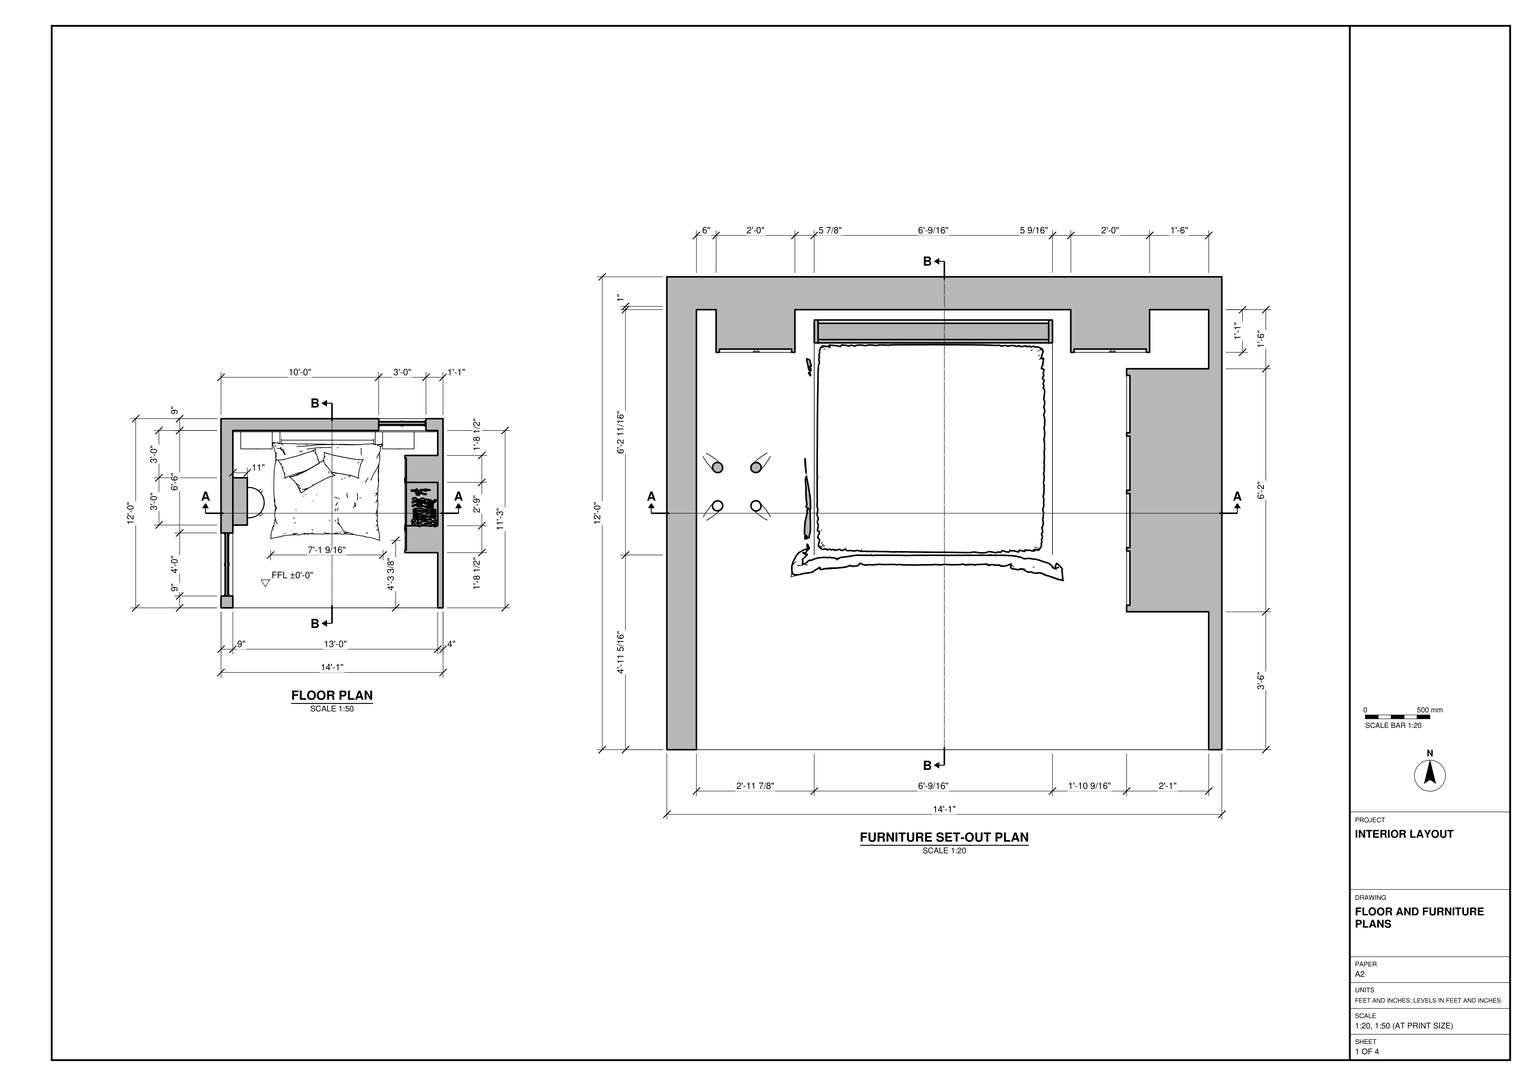
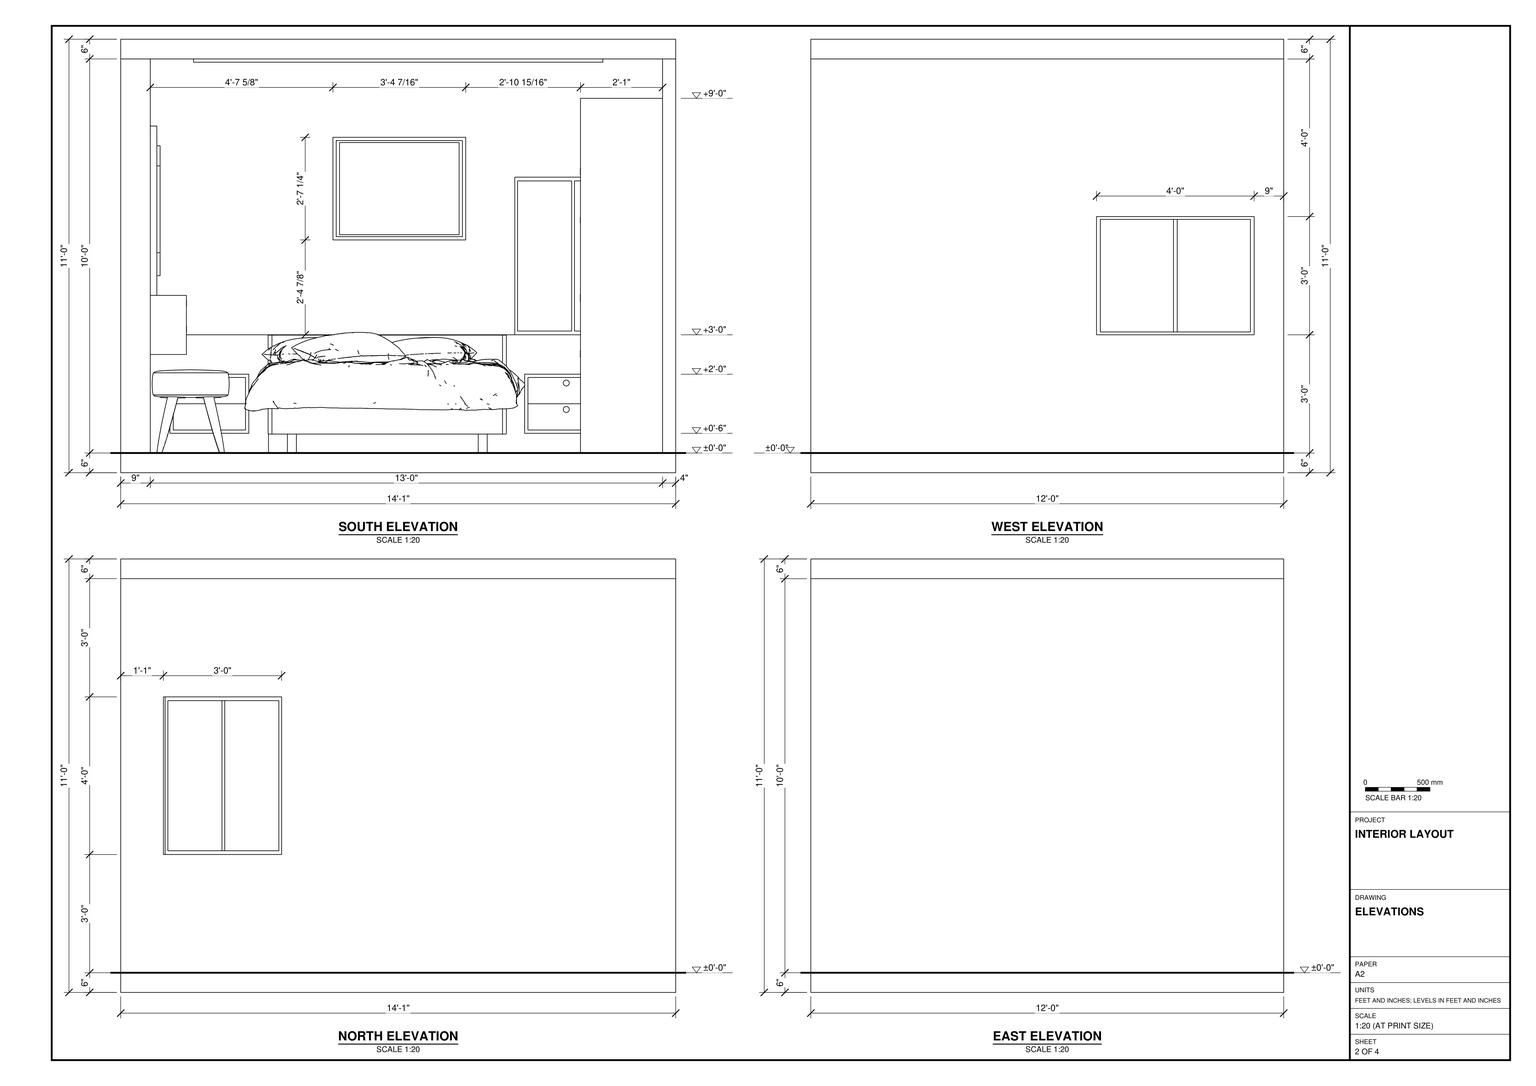
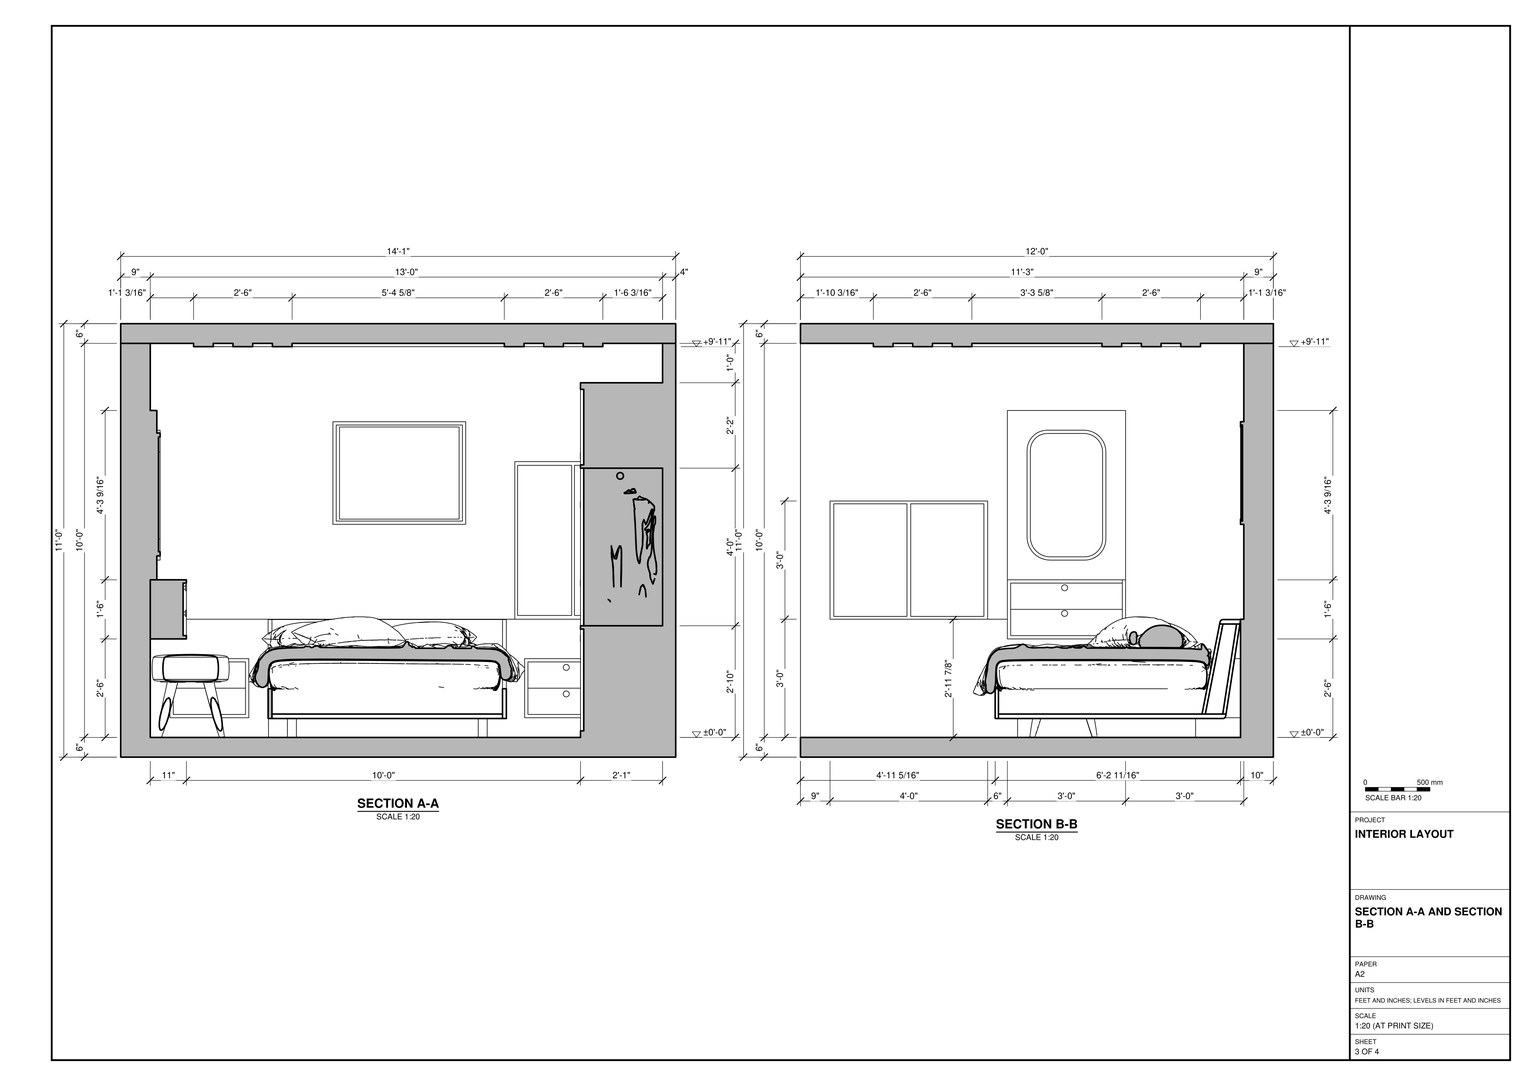
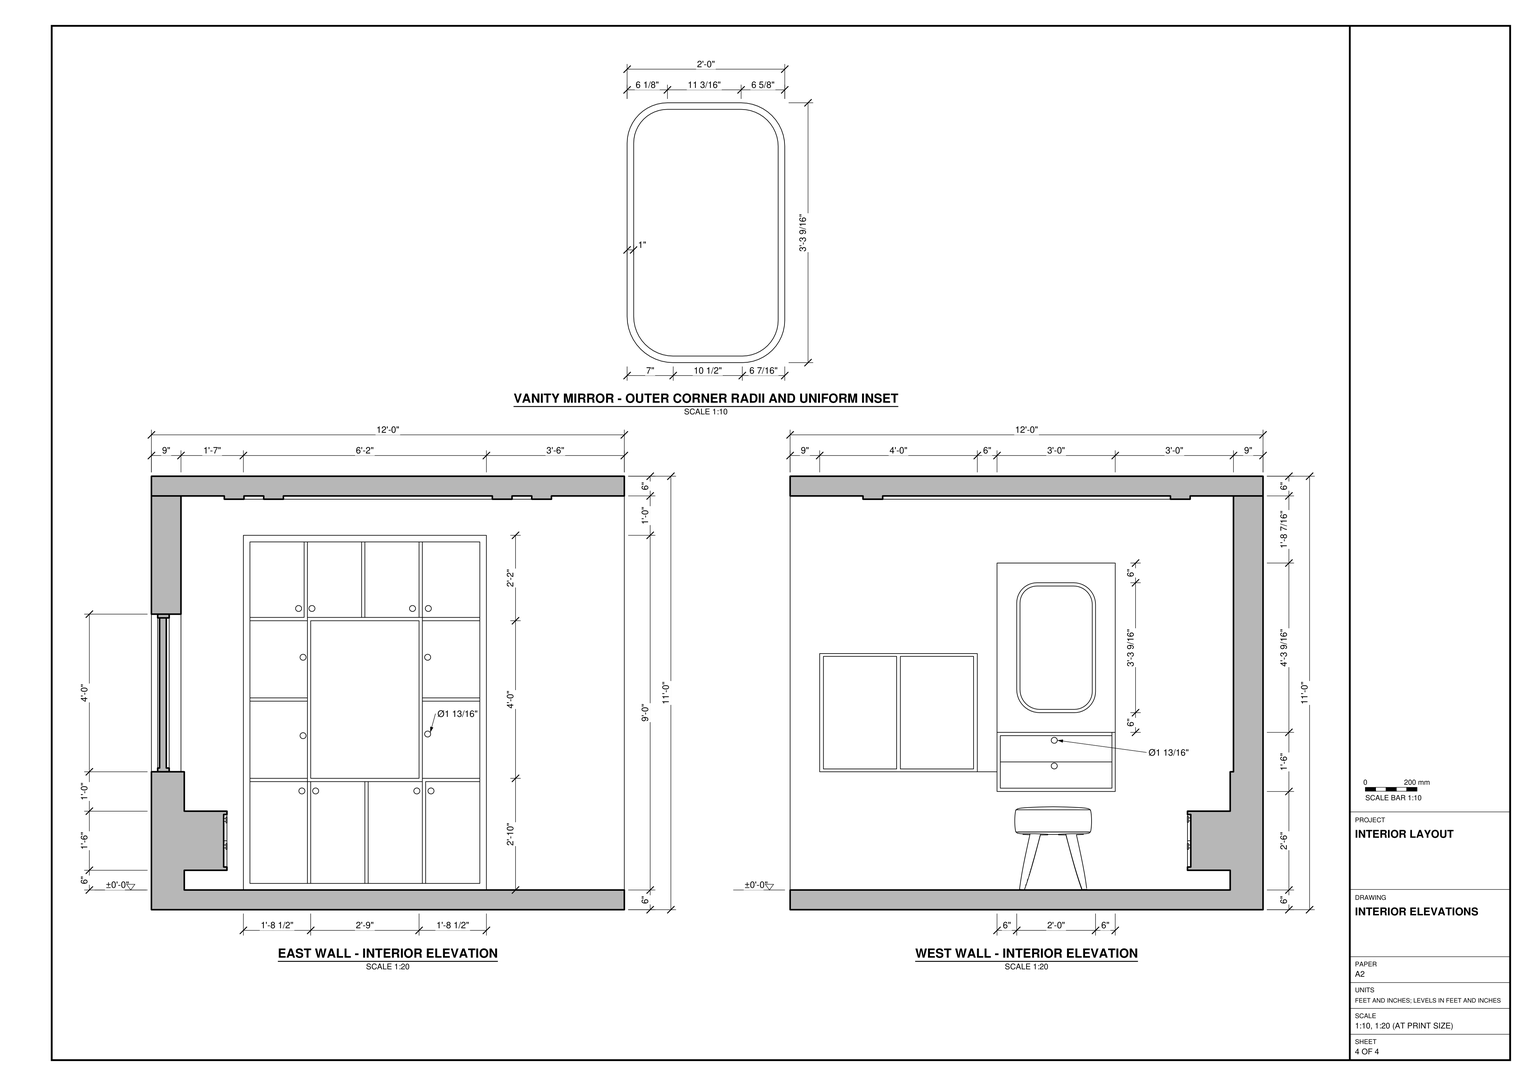
Build the bedroom shown in task_files/diagram_01.pdf in SketchUp. Work in feet and inches. The room shell measures 14'-1" east to west, 12'-0" north to south and 11'-0" overall in height. Set the finished floor at ±0'-0". Model the 6" floor and ceiling slabs with 10'-0" clear between them. Leave the south side open as drawn. Make the north and west walls 9" thick and the east wall 4" thick. Fit divided window units in the north and west wall openings, using the elevations to distinguish the taller north window from the wider west window.

Use the furniture set-out plan to position the bed with its headboard against the north wall and a bedside drawer unit on either side. Place the framed item above the bed. Model the wardrobe along the east wall, including the hanging compartment shown in section. On the west wall, place the shallow dressing unit beside the window, with its mirror above and stool in front. Decor and loose items may be any suitable library components placed as shown.

Keep the walls, slabs and individual furniture and joinery pieces in separate groups or components, and use components for repeated parts. Save one SketchUp model as output_files/bedroom_with_fitted_storage_and_a_dressing_area.skp.

# SketchUp Ruby script. Lengths in inches.
U = 1.inch
M = Sketchup.active_model
def pt(a) = Geom::Point3d.new(a.map { |v| v * U })
def face(e, loops, mat)
  f = e.add_face(loops[0].map { |a| pt(a) })
  loops[1..].each { |l| e.add_face(l.map { |a| pt(a) }).erase! }
  f.material = f.back_material = mat if mat
  f
end
# faces: each face lists its corners as indices into pts; further lists are holes
def faces(e, pts, list, mat = nil) = list.each { |f| face(e, (f[0].is_a?(Array) ? f : [f]).map { |l| l.map { |i| pts[i] } }, mat) }
# xy, xz, yz: faces in a plane at the given z, y or x. An outline is a flat list of corners, or four numbers for a rectangle; further outlines are holes
def ring(l) = l.size == 4 ? [[l[0], l[1]], [l[2], l[1]], [l[2], l[3]], [l[0], l[3]]] : l.each_slice(2).to_a
def flat(e, list, mat, &to3) = list.each { |f| face(e, (f[0].is_a?(Array) ? f : [f]).map { |l| ring(l).map { |u, v| to3.(u, v) } }, mat) }
def xy(e, z, list, mat = nil) = flat(e, list, mat) { |x, y| [x, y, z] }
def xz(e, y, list, mat = nil) = flat(e, list, mat) { |x, z| [x, y, z] }
def yz(e, x, list, mat = nil) = flat(e, list, mat) { |y, z| [x, y, z] }
def lines(e, pts, list) = list.each { |a, b| e.add_line(pt(pts[a]), pt(pts[b])) }
# prism: a flat outline (further loops are holes) pulled along v
def prism(e, loops, v, mat = nil)
  f = face(e, loops, mat); d = Geom::Vector3d.new(v.map { |x| x * U })
  f.pushpull(f.normal.samedirection?(d) ? d.length : -d.length)
end
def box(e, o, s, mat = nil) = prism(e, [[o, [o[0] + s[0], o[1], o[2]], [o[0] + s[0], o[1] + s[1], o[2]], [o[0], o[1] + s[1], o[2]]]], [0, 0, s[2]], mat)
def at(x, y, z, deg = 0) = Geom::Transformation.translation(pt([x, y, z])) * Geom::Transformation.rotation(ORIGIN, Z_AXIS, deg.degrees)
def axes(o, x, y, z) = Geom::Transformation.new([*x, 0, *y, 0, *z, 0, *pt(o).to_a, 1])
def part(name) = M.definitions.add(name)
# library, detail: a bought-in or finely detailed component or shape, given as its bounding box
def library(name, o, s) = part(name).tap { |d| box(d.entities, o, s) }
def detail(e, o, s) = box(e.add_group.entities, o, s)
def put(e, d, t, mat = nil) = e.add_instance(d, t).tap { |i| i.material = mat if mat }
def group(e, t, mat = nil) = e.add_group.tap { |g| g.transformation = t; g.material = mat if mat }.entities
root = M.entities
M.materials.add("F4").color = [207, 206, 198]
M.materials.add("Querkus Oak Naturel Adagio _ Architonic1").color = [173, 130, 81]
M.materials.add("[0052_FloralWhite]").color = [255, 250, 240]
M.materials.add("[Carrera Marble]").color = [207, 207, 207]
M.materials.add("[Color M09]4").color = [0, 0, 0]
M.materials.add("[Color_008]").color = [30, 30, 30]
M.materials.add("[Color_009]").color = [0, 0, 0]
M.materials.add("[Formica Laminate Light]").color = [213, 189, 164]
M.materials.add("[Mirror 02]").color = [234, 234, 223]
M.materials.add("[Translucent Glass Blue]1").color = [255, 255, 255]
M.materials["[Translucent Glass Blue]1"].alpha = 0.5
M.materials.add("[Translucent_Glass_Gray]1").color = [128, 128, 128]
M.materials["[Translucent_Glass_Gray]1"].alpha = 0.5
M.materials.add("[Wood Veneer 01]").color = [120, 70, 37]
c1 = library("BED+04",[-44.14,-47.125,0],[86.23,97.52,31.95])
c2 = library("男襯衫(短)+女風衣2件",[-14.24,-20.45,6.32],[25.88,57.24,61.83])
c3 = library("Group115\#1",[-65.86,-17.6875,-11.76],[68.92,35.16,52.98])
c4 = library("stool",[-0.68,-0.68,0],[1.36,1.36,1.75])
c5 = part("Janela (3)")
xy(c5.entities,0,[[96.33,43.17,179.01,44.35]],"[Color_009]")
xy(c5.entities,1.97,[[98.3,44.15,136.6875,44.35],[138.66,44.15,177.04,44.35]])
xy(c5.entities,1.97,[[98.3,43.17,136.6875,43.46],[138.66,43.17,177.04,43.46]],"[Color_009]")
xy(c5.entities,80.71,[[98.3,43.17,136.6875,43.46],[138.66,43.17,177.04,43.46],[98.3,43.46,136.6875,44.15],[138.66,43.46,177.04,44.15],[98.3,44.15,136.6875,44.35],
  [138.66,44.15,177.04,44.35]])
xy(c5.entities,82.68,[[96.33,43.17,179.01,44.35]],"[Color_008]")
xz(c5.entities,43.17,[[[96.33,0,179.01,82.68],[98.3,1.97,136.6875,80.71],[138.66,1.97,177.04,80.71]]],"[Color_009]")
xz(c5.entities,43.46,[[98.3,1.97,136.6875,80.71],[138.66,1.97,177.04,80.71]],"[Translucent_Glass_Gray]1")
xz(c5.entities,44.15,[[98.3,1.97,136.6875,80.71],[138.66,1.97,177.04,80.71]],"[Translucent_Glass_Gray]1")
xz(c5.entities,44.35,[[[96.33,0,179.01,82.68],[98.3,1.97,177.04,80.71]],[136.6875,1.97,138.66,80.71]],"[Color_009]")
yz(c5.entities,96.33,[[43.17,0,44.35,82.68]],"[Color_009]")
yz(c5.entities,98.3,[[44.15,1.97,44.35,80.71]])
yz(c5.entities,98.3,[[43.17,1.97,43.46,80.71]],"[Color_009]")
yz(c5.entities,136.6875,[[43.17,1.97,43.46,80.71],[44.15,1.97,44.35,80.71]],"[Color_009]")
yz(c5.entities,138.66,[[43.17,1.97,43.46,80.71],[44.15,1.97,44.35,80.71]])
yz(c5.entities,177.04,[[43.17,1.97,43.46,80.71],[44.15,1.97,44.35,80.71]],"[Color_009]")
yz(c5.entities,179.01,[[43.17,0,44.35,82.68]],"[Color_009]")
c6 = part("Handle+Collection")
g1 = group(c6.entities,at(29.7,-26.29,-4.18))
xz(g1,0,[[-0.79,-1.58,-0.59,-1.55,-0.4,-1.48,-0.23,-1.35,-0.11,-1.1875,-0.03,-1,0,-0.79,-0.03,-0.59,-0.11,-0.4,-0.23,-0.23,-0.4,-0.11,-0.59,-0.03,-0.79,0,-1,-0.03,-1.1875,-0.11,-1.35,-0.23,-1.48,-0.4,-1.55,-0.59,-1.58,-0.79,-1.55,-1,-1.48,-1.1875,-1.35,-1.35,-1.1875,-1.48,-1,-1.55]],"[Color M09]4")
xz(g1,0.39,[[[-0.79,-1.58,-1,-1.55,-1.1875,-1.48,-1.35,-1.35,-1.48,-1.1875,-1.55,-1,-1.58,-0.79,-1.55,-0.59,-1.48,-0.4,-1.35,-0.23,-1.1875,-0.11,-1,-0.03,-0.79,0,-0.59,-0.03,-0.4,-0.11,-0.23,-0.23,-0.11,-0.4,-0.03,-0.59,0,-0.79,-0.03,-1,-0.11,-1.1875,-0.23,-1.35,-0.4,-1.48,-0.59,-1.55],[-0.79,-1.18,-0.6875,-1.17,-0.59,-1.13,-0.51,-1.07,-0.45,-0.99,-0.41,-0.89,-0.4,-0.79,-0.41,-0.6875,-0.45,-0.59,-0.51,-0.51,-0.59,-0.45,-0.6875,-0.41,-0.79,-0.4,-0.89,-0.41,-0.99,-0.45,-1.07,-0.51,-1.13,-0.59,-1.17,-0.6875,-1.18,-0.79,-1.17,-0.89,-1.13,-0.99,-1.07,-1.07,-0.99,-1.13,-0.89,-1.17]]],"[Color M09]4")
p = [[-1.1875,0.39,-1.48],[-1,0.39,-1.55],[-1,0,-1.55],[-1.1875,0,-1.48],[-0.79,0.39,-1.58],[-0.79,0,-1.58],
  [-0.59,0.39,-1.55],[-0.59,0,-1.55],[-0.4,0.39,-1.48],[-0.4,0,-1.48],[-1.35,0.39,-1.35],[-1.35,0,-1.35],
  [-0.23,0.39,-1.35],[-0.23,0,-1.35],[-1.48,0.39,-1.1875],[-1.48,0,-1.1875],[-0.11,0.39,-1.1875],[-0.11,0,-1.1875],
  [-1.55,0.39,-1],[-1.55,0,-1],[-0.03,0.39,-1],[-0.03,0,-1],[-0.99,1.18,-1.13],[-0.89,1.18,-1.17],
  [-0.89,0.39,-1.17],[-0.99,0.39,-1.13],[-0.79,1.18,-1.18],[-0.79,0.39,-1.18],[-0.6875,1.18,-1.17],[-0.6875,0.39,-1.17],
  [-0.59,1.18,-1.13],[-0.59,0.39,-1.13],[-1.07,1.18,-1.07],[-1.07,0.39,-1.07],[-1.13,1.18,-0.99],[-1.13,0.39,-0.99],
  [-0.51,1.18,-1.07],[-0.51,0.39,-1.07],[-0.45,1.18,-0.99],[-0.45,0.39,-0.99],[-1.58,0.39,-0.79],[-1.58,0,-0.79],
  [0,0.39,-0.79],[0,0,-0.79],[-1.17,1.18,-0.89],[-1.17,0.39,-0.89],[-0.41,1.18,-0.89],[-0.41,0.39,-0.89],
  [-1.18,1.18,-0.79],[-1.18,0.39,-0.79],[-0.4,1.18,-0.79],[-0.4,0.39,-0.79],[-1.55,0.39,-0.59],[-1.55,0,-0.59],
  [-0.03,0.39,-0.59],[-0.03,0,-0.59],[-1.17,1.18,-0.6875],[-1.17,0.39,-0.6875],[-0.41,1.18,-0.6875],[-0.41,0.39,-0.6875],
  [-1.13,1.18,-0.59],[-1.13,0.39,-0.59],[-0.45,1.18,-0.59],[-0.45,0.39,-0.59],[-1.48,0.39,-0.4],[-1.48,0,-0.4],
  [-0.11,0.39,-0.4],[-0.11,0,-0.4],[-1.07,1.18,-0.51],[-1.07,0.39,-0.51],[-0.51,1.18,-0.51],[-0.51,0.39,-0.51],
  [-0.99,1.18,-0.45],[-0.99,0.39,-0.45],[-0.59,1.18,-0.45],[-0.59,0.39,-0.45],[-1.35,0.39,-0.23],[-1.35,0,-0.23],
  [-0.23,0.39,-0.23],[-0.23,0,-0.23],[-0.89,1.18,-0.41],[-0.89,0.39,-0.41],[-0.79,1.18,-0.4],[-0.79,0.39,-0.4],
  [-0.6875,1.18,-0.41],[-0.6875,0.39,-0.41],[-1.1875,0.39,-0.11],[-1.1875,0,-0.11],[-0.4,0.39,-0.11],[-0.4,0,-0.11],
  [-1,0.39,-0.03],[-1,0,-0.03],[-0.59,0.39,-0.03],[-0.59,0,-0.03],[-0.79,0.39,0],[-0.79,0,0]]
faces(g1,p,[[0,1,2,3],[1,4,5,2],[4,6,7,5],[6,8,9,7],[10,0,3,11],[8,12,13,9],[14,10,11,15],[12,16,17,13],
  [18,14,15,19],[16,20,21,17],[22,23,24,25],[23,26,27,24],[26,28,29,27],[28,30,31,29],[32,22,25,33],[34,32,33,35],
  [30,36,37,31],[36,38,39,37],[40,18,19,41],[20,42,43,21],[44,34,35,45],[38,46,47,39],[48,44,45,49],[46,50,51,47],
  [52,40,41,53],[42,54,55,43],[56,48,49,57],[50,58,59,51],[60,56,57,61],[58,62,63,59],[64,52,53,65],[54,66,67,55],
  [68,60,61,69],[62,70,71,63],[72,68,69,73],[70,74,75,71],[76,64,65,77],[66,78,79,67],[80,72,73,81],[82,80,81,83],
  [84,82,83,85],[74,84,85,75],[86,76,77,87],[78,88,89,79],[90,86,87,91],[88,92,93,89],[94,90,91,95],[92,94,95,93]],"[Color M09]4")
c7 = part("F2")
g2 = group(c7.entities,at(24,0,0))
xy(g2,0.5,[[0.5,0.3,18.5,0.6]])
xy(g2,24,[[0.5,0.3,18.5,0.6]])
xz(g2,0.3,[[0.5,0.5,18.5,24]],"F4")
xz(g2,0.6,[[0.5,0.5,18.5,24]])
yz(g2,0.5,[[0.3,0.5,0.6,24]])
yz(g2,18.5,[[0.3,0.5,0.6,24]])
g3 = group(g2,at(0,0,0),"Querkus Oak Naturel Adagio _ Architonic1")
prism(g3,[[[0,0.6,0],[0,0.6,24.5],[19,0.6,24.5],[19,0.6,0]],[[0.5,0.6,0.5],[18.5,0.6,0.5],[18.5,0.6,24],[0.5,0.6,24]]],[0,-0.6,0])
put(root,c1,axes([81.56,91.3,6],[0.99247,0,0],[0,0.84715,0],[0,0,1.15]))
put(root,c2,axes([153.08,88.11,35.1875],[0.76,0,0],[0,0.21607,0],[0,0,0.76121]))
put(root,c3,axes([154.78,83.54,54.44],[0,0.34098,0],[-0.57761,0,0],[0,0,0.8]))
put(root,c4,axes([21.3,80.09,6],[17.325,0,0],[0,17.278,0],[0,0,14.4752]))
put(root,c5,axes([78.65,10.82,42],[0.42922,0,0],[0,2.96,0],[0,0,0.58057]))
put(root,c5,axes([122.28,-46.93,42],[0,0.58057,0],[-2.6936,0,0],[0,0,0.43543]))
put(root,c6,axes([163.34,93.41,97.46],[0,-1.16636,0],[0.88985,0,0],[0,0,1.15358]))
put(root,c6,axes([163.34,98.22,97.46],[0,-1.16636,0],[0.88985,0,0],[0,0,1.15358]))
put(root,c6,axes([163.34,128.85,97.46],[0,-1.16636,0],[0.88985,0,0],[0,0,1.15358]))
put(root,c6,axes([163.34,132.91,97.46],[0,-1.16636,0],[0.88985,0,0],[0,0,1.15358]))
put(root,c6,axes([163.34,131.91,41.9],[0,-1.16636,0],[0.88985,0,0],[0,0,1.15358]))
put(root,c6,axes([163.34,127.72,41.9],[0,-1.16636,0],[0.88985,0,0],[0,0,1.15358]))
put(root,c6,axes([163.34,96.91,41.9],[0,-1.16636,0],[0.88985,0,0],[0,0,1.15358]))
put(root,c6,axes([163.34,92.6,41.9],[0,-1.16636,0],[0.88985,0,0],[0,0,1.15358]))
put(root,c6,axes([163.35,93.61,59.23],[0,-1.16636,0],[0.88985,0,0],[0,0,1.15358]))
put(root,c6,axes([163.35,93.61,82.61],[0,-1.16636,0],[0.88985,0,0],[0,0,1.15358]))
put(root,c6,axes([163.35,131.55,82.61],[0,-1.16636,0],[0.88985,0,0],[0,0,1.15358]))
put(root,c6,axes([163.35,131.55,58.73],[0,-1.16636,0],[0.88985,0,0],[0,0,1.15358]))
put(root,c6,axes([-3.35,46.7,57.32],[0,1.16636,0],[-0.88985,0,0],[0,0,1.15358]))
put(root,c6,axes([-6.49,144.35,33.24],[1.16636,0,0],[0,0.88985,0],[0,0,1.15358]))
put(root,c6,axes([-6.49,144.35,24.99],[1.16636,0,0],[0,0.88985,0],[0,0,1.15358]))
put(root,c6,axes([101.95,144.35,24.99],[1.16636,0,0],[0,0.88985,0],[0,0,1.15358]))
put(root,c6,axes([101.95,144.35,33.05],[1.16636,0,0],[0,0.88985,0],[0,0,1.15358]))
put(root,c6,axes([-3.35,46.7,49.51],[0,1.16636,0],[-0.88985,0,0],[0,0,1.15358]))
g4 = group(root,at(0,0,0),"[0052_FloralWhite]")
xy(g4,0,[[0,0,169,144]],"[0052_FloralWhite]")
xy(g4,6,[[9,0,165,0,165,42,140,42,140,116,165,116,165,134,9,134]],"[Carrera Marble]")
xy(g4,8,[[140,44,141,60.5],[140,61.5,141,78],[140,79,141,95.5],[140,96.5,141,114]],"[Wood Veneer 01]")
xy(g4,12,[[123,121,147,134]])
xy(g4,12,[[15,121,39,134]],"[Wood Veneer 01]")
xy(g4,13,[[16,121,38,122],[124,121,146,122]],"[Wood Veneer 01]")
xy(g4,29,[[16,121,38,122],[124,121,146,122]],"[Wood Veneer 01]")
xy(g4,30,[[15,121,39,134],[123,121,147,134]],"[Wood Veneer 01]")
xy(g4,36,[[9,63,20,99]],"[Formica Laminate Light]")
xy(g4,37,[[19,64,20,98]],"[Formica Laminate Light]")
xy(g4,39,[[140,44,141,60.5],[140,61.5,141,78],[140,79,141,95.5],[140,96.5,141,114]],"[Wood Veneer 01]")
xy(g4,40,[[141,62.5,165,95.5]])
xy(g4,40,[[140,44,141,61.5],[140,62.5,141,95.5],[140,96.5,141,114]],"[Wood Veneer 01]")
xy(g4,42,[[0,9,9,57],[120,135,156,144]],"[0052_FloralWhite]")
xy(g4,42,[[9,134,165,135]],"[Wood Veneer 01]")
xy(g4,53,[[19,64,20,98]],"[Formica Laminate Light]")
xy(g4,54,[[9,63,11,64],[9,64,11,98],[9,98,11,99]])
xy(g4,54,[[11,63,20,99]],"[Formica Laminate Light]")
xy(g4,60,[[11,76.02,12,86.54]])
xy(g4,61,[[11.5,76.02,12,86.54]],"[Wood Veneer 01]")
xy(g4,63.5,[[140,44,141,61.5],[140,96.5,141,114]],"[Wood Veneer 01]")
xy(g4,64.5,[[140,44,141,61.5],[140,96.5,141,114]],"[Wood Veneer 01]")
xy(g4,70.89,[[64.62,134,105.06,135]],"[Wood Veneer 01]")
xy(g4,71.89,[[65.62,134,104.06,134.5]],"[Wood Veneer 01]")
xy(g4,78,[[0,9,9,57]],"[0052_FloralWhite]")
xy(g4,84.66,[[151.97,62.5,152.03,95.5],[152.16,62.5,152.22,95.5]])
xy(g4,86.65,[[152.01,62.5,152.08,95.5],[152.08,62.5,152.14,95.5],[152.14,62.5,152.2,95.5]])
xy(g4,88,[[141,62.5,165,95.5]])
xy(g4,88,[[140,44,141,61.5],[140,62.5,141,95.5],[140,96.5,141,114]],"[Wood Veneer 01]")
xy(g4,89,[[140,44,141,61.5],[140,62.5,141,79],[140,80,141,96.5],[140,97.5,141,114]],"[Wood Veneer 01]")
xy(g4,90,[[120,135,156,144]],"[0052_FloralWhite]")
xy(g4,98.5625,[[11.5,75.14,12,86.35]],"[Wood Veneer 01]")
xy(g4,99.5625,[[11,75.14,12,86.35]],"[Wood Veneer 01]")
xy(g4,101.14,[[65.62,134,104.06,134.5]],"[Wood Veneer 01]")
xy(g4,102.14,[[64.62,134,105.06,135]],"[Wood Veneer 01]")
xy(g4,105.5625,[[9,63,11,99]],"[Formica Laminate Light]")
xy(g4,112,[[140,44,141,61.5],[140,62.5,141,79],[140,80,141,96.5],[140,97.5,141,114]],"[Wood Veneer 01]")
xy(g4,114,[[140,42,165,116]],"[Wood Veneer 01]")
xy(g4,126,[[0,0,9,0,9,135,165,135,165,134,169,134,169,144,0,144],[165,0,169,134]])
xz(g4,0,[[0,0,169,0,169,126,165,126,165,6,9,6,9,126,0,126]],"[0052_FloralWhite]")
xz(g4,9,[[0,42,9,78]],"[0052_FloralWhite]")
xz(g4,42,[[140,6,165,114]],"[Wood Veneer 01]")
xz(g4,44,[[140,8,141,39],[140,40,141,63.5],[140,64.5,141,88],[140,89,141,112]],"[Wood Veneer 01]")
xz(g4,57,[[0,42,9,78]],"[0052_FloralWhite]")
xz(g4,60.5,[[140,8,141,39]],"[Wood Veneer 01]")
xz(g4,61.5,[[140,8,141,39],[140,40,141,63.5],[140,64.5,141,88],[140,89,141,112]],"[Wood Veneer 01]")
xz(g4,62.5,[[[141,40,165,88],[152.1,84.65,152.16,84.66,152.22,84.66,152.28,84.67,152.35,84.6875,152.41,84.71,152.46,84.73,152.52,84.75,152.58,84.78,152.63,84.82,152.68,84.85,152.78,84.93,152.9,85.08,152.9375,85.13,152.97,85.18,153,85.24,153.06,85.42,153.08,85.54,153.08,85.6,153.09,85.67,153.08,85.73,153.08,85.79,153.07,85.85,152.99,86.09,152.96,86.15,152.92,86.2,152.89,86.25,152.81,86.35,152.76,86.39,152.72,86.43,152.67,86.47,152.61,86.5,152.56,86.54,152.5,86.5625,152.44,86.59,152.38,86.61,152.26,86.64,152.2,86.65,152.01,86.65,151.83,86.62,151.71,86.58,151.59,86.52,151.49,86.46,151.44,86.42,151.39,86.375,151.35,86.33,151.27,86.23,151.24,86.18,151.2,86.125,151.18,86.07,151.15,86.01,151.13,85.95,151.12,85.89,151.1,85.83,151.09,85.77,151.09,85.58,151.11,85.46,151.12,85.39,151.14,85.33,151.16,85.28,151.1875,85.22,151.22,85.16,151.28,85.06,151.32,85.01,151.41,84.92,151.46,84.875,151.51,84.84,151.56,84.8,151.61,84.77,151.67,84.74,151.85,84.68,151.97,84.66,152.03,84.66]]])
xz(g4,62.5,[[140,40,141,88],[140,89,141,112]],"[Wood Veneer 01]")
xz(g4,63,[[9,36,20,54],[9,54,11,105.5625]],"[Formica Laminate Light]")
xz(g4,64,[[19,37,20,53]],"[Formica Laminate Light]")
xz(g4,69,[[11,67.02,12,93.42]],"[Wood Veneer 01]")
xz(g4,70,[[11.5,67.02,12,93.42]],"[Wood Veneer 01]")
xz(g4,78,[[140,8,141,39]],"[Wood Veneer 01]")
xz(g4,79,[[140,8,141,39],[140,89,141,112]],"[Wood Veneer 01]")
xz(g4,80,[[140,89,141,112]],"[Wood Veneer 01]")
xz(g4,92,[[11.5,66.46,12,92.91]],"[Wood Veneer 01]")
xz(g4,93,[[11,66.46,12,92.91]],"[Wood Veneer 01]")
xz(g4,95.5,[[[141,40,165,88],[152.1,84.65,152.03,84.66,151.97,84.66,151.85,84.68,151.67,84.74,151.61,84.77,151.56,84.8,151.51,84.84,151.46,84.875,151.41,84.92,151.32,85.01,151.28,85.06,151.22,85.16,151.1875,85.22,151.16,85.28,151.14,85.33,151.12,85.39,151.11,85.46,151.09,85.58,151.09,85.77,151.1,85.83,151.12,85.89,151.13,85.95,151.15,86.01,151.18,86.07,151.2,86.125,151.24,86.18,151.27,86.23,151.35,86.33,151.39,86.375,151.44,86.42,151.49,86.46,151.59,86.52,151.71,86.58,151.83,86.62,152.01,86.65,152.2,86.65,152.26,86.64,152.38,86.61,152.44,86.59,152.5,86.5625,152.56,86.54,152.61,86.5,152.67,86.47,152.72,86.43,152.76,86.39,152.81,86.35,152.89,86.25,152.92,86.2,152.96,86.15,152.99,86.09,153.07,85.85,153.08,85.79,153.08,85.73,153.09,85.67,153.08,85.6,153.08,85.54,153.06,85.42,153,85.24,152.97,85.18,152.9375,85.13,152.9,85.08,152.78,84.93,152.68,84.85,152.63,84.82,152.58,84.78,152.52,84.75,152.46,84.73,152.41,84.71,152.35,84.6875,152.28,84.67,152.22,84.66,152.16,84.66]]])
xz(g4,95.5,[[140,8,141,39],[140,40,141,88]],"[Wood Veneer 01]")
xz(g4,96.5,[[140,8,141,39],[140,40,141,63.5],[140,64.5,141,88],[140,89,141,112]],"[Wood Veneer 01]")
xz(g4,97.5,[[140,89,141,112]],"[Wood Veneer 01]")
xz(g4,98,[[19,37,20,53]],"[Formica Laminate Light]")
xz(g4,99,[[9,36,20,54],[9,54,11,105.5625]],"[Formica Laminate Light]")
xz(g4,114,[[140,8,141,39],[140,40,141,63.5],[140,64.5,141,88],[140,89,141,112]],"[Wood Veneer 01]")
xz(g4,116,[[140,6,165,114]],"[Wood Veneer 01]")
xz(g4,121,[[[15,12,39,30],[16,13,38,29]],[[123,12,147,30],[124,13,146,29]]],"[Wood Veneer 01]")
xz(g4,122,[[16,13,38,21],[124,13,146,21],[16,21,38,29],[124,21,146,29]],"[Wood Veneer 01]")
xz(g4,134,[[[9,6,165,42],[123,12,147,30],[15,12,39,30]],[[64.62,70.89,105.06,102.14],[65.62,71.89,104.06,101.14]]],"[Wood Veneer 01]")
xz(g4,134.5,[[65.62,71.89,104.06,101.14]],"[0052_FloralWhite]")
xz(g4,135,[[[9,42,120,42,120,90,156,90,156,42,165,42,165,126,9,126],[64.62,70.89,105.06,102.14]]],"[0052_FloralWhite]")
xz(g4,144,[[[0,0,169,126],[120,42,156,90]]],"[0052_FloralWhite]")
yz(g4,0,[[[0,0,144,126],[9,42,57,78]]],"[0052_FloralWhite]")
yz(g4,9,[[63,36,99,54]])
yz(g4,9,[[[0,6,134,6,134,42,135,42,135,126,0,126],[63,36,63,42,9,42,9,78,57,78,57,42,63,42,63,105.5625,99,105.5625,99,36]]],"[0052_FloralWhite]")
yz(g4,11,[[[63,54,99,105.5625],[76.02,60,75.1,60.06,74.2,60.24,73.33,60.53,72.51,60.94,71.75,61.45,71.06,62.06,70.45,62.75,69.94,63.51,69.53,64.33,69.24,65.2,69.06,66.1,69,67.02,69,93.42,69.05,94.22,69.21,95.01,69.47,95.77,69.82,96.49,70.27,97.16,70.8,97.76,71.4,98.29,72.07,98.74,72.79,99.09,73.55,99.35,74.34,99.51,75.14,99.5625,86.35,99.5625,87.22,99.5,88.07,99.34,88.9,99.06,89.68,98.67,90.4,98.1875,91.05,97.61,91.625,96.96,92.11,96.24,92.49,95.46,92.77,94.63,92.94,93.78,93,92.91,93,66.46,92.94,65.62,92.78,64.79,92.51,63.99,92.13,63.23,91.66,62.53,91.11,61.89,90.47,61.34,89.77,60.87,89.01,60.49,88.21,60.22,87.38,60.06,86.54,60]]],"[Formica Laminate Light]")
yz(g4,11.5,[[76.02,61,86.54,61,87.25,61.05,87.95,61.1875,88.63,61.42,89.27,61.73,89.86,62.13,90.4,62.6,90.87,63.14,91.27,63.73,91.58,64.37,91.8125,65.05,91.95,65.75,92,66.46,92,92.91,91.95,93.65,91.81,94.375,91.57,95.08,91.24,95.74,90.83,96.35,90.35,96.91,89.79,97.39,89.18,97.81,88.51,98.13,87.8125,98.37,87.09,98.51,86.35,98.5625,75.14,98.5625,74.47,98.52,73.81,98.39,73.17,98.17,72.57,97.875,72.01,97.5,71.51,97.06,71.0625,96.55,70.6875,95.99,70.39,95.39,70.18,94.75,70.04,94.09,70,93.42,70,67.02,70.05,66.23,70.21,65.46,70.46,64.71,70.81,64.01,71.24,63.35,71.76,62.76,72.35,62.24,73.01,61.81,73.71,61.46,74.46,61.21,75.23,61.05]],"[Mirror 02]")
yz(g4,12,[[[76.02,60,86.54,60,87.38,60.06,88.21,60.22,89.01,60.49,89.77,60.87,90.47,61.34,91.11,61.89,91.66,62.53,92.13,63.23,92.51,63.99,92.78,64.79,92.94,65.62,93,66.46,93,92.91,92.94,93.78,92.77,94.63,92.49,95.46,92.11,96.24,91.625,96.96,91.05,97.61,90.4,98.1875,89.68,98.67,88.9,99.06,88.07,99.34,87.22,99.5,86.35,99.5625,75.14,99.5625,74.34,99.51,73.55,99.35,72.79,99.09,72.07,98.74,71.4,98.29,70.8,97.76,70.27,97.16,69.82,96.49,69.47,95.77,69.21,95.01,69.05,94.22,69,93.42,69,67.02,69.06,66.1,69.24,65.2,69.53,64.33,69.94,63.51,70.45,62.75,71.06,62.06,71.75,61.45,72.51,60.94,73.33,60.53,74.2,60.24,75.1,60.06],[76.02,61,75.23,61.05,74.46,61.21,73.71,61.46,73.01,61.81,72.35,62.24,71.76,62.76,71.24,63.35,70.81,64.01,70.46,64.71,70.21,65.46,70.05,66.23,70,67.02,70,93.42,70.04,94.09,70.18,94.75,70.39,95.39,70.6875,95.99,71.0625,96.55,71.51,97.06,72.01,97.5,72.57,97.875,73.17,98.17,73.81,98.39,74.47,98.52,75.14,98.5625,86.35,98.5625,87.09,98.51,87.8125,98.37,88.51,98.13,89.18,97.81,89.79,97.39,90.35,96.91,90.83,96.35,91.24,95.74,91.57,95.08,91.81,94.375,91.95,93.65,92,92.91,92,66.46,91.95,65.75,91.8125,65.05,91.58,64.37,91.27,63.73,90.87,63.14,90.4,62.6,89.86,62.13,89.27,61.73,88.63,61.42,87.95,61.1875,87.25,61.05,86.54,61]]],"[Wood Veneer 01]")
yz(g4,15,[[121,12,134,30]],"[Wood Veneer 01]")
yz(g4,16,[[121,13,122,21],[121,21,122,29]],"[Wood Veneer 01]")
yz(g4,19,[[64,37,98,45],[64,45,98,53]],"[Formica Laminate Light]")
yz(g4,20,[[63,36,99,36,99,54,98,54,98,37,64,37,64,53,98,53,98,54,63,54]],"[Formica Laminate Light]")
yz(g4,38,[[121,13,122,21],[121,21,122,29]],"[Wood Veneer 01]")
yz(g4,39,[[121,12,134,30]],"[Wood Veneer 01]")
yz(g4,64.62,[[134,70.89,135,102.14]],"[Wood Veneer 01]")
yz(g4,65.62,[[134,71.89,134.5,101.14]],"[Wood Veneer 01]")
yz(g4,104.06,[[134,71.89,134.5,101.14]],"[Wood Veneer 01]")
yz(g4,105.06,[[134,70.89,135,102.14]],"[Wood Veneer 01]")
yz(g4,120,[[135,42,144,90]],"[0052_FloralWhite]")
yz(g4,123,[[121,12,134,30]],"[Wood Veneer 01]")
yz(g4,124,[[121,13,122,21],[121,21,122,29]],"[Wood Veneer 01]")
yz(g4,140,[[[42,6,116,114],[44,8,114,112]],[60.5,8,60.5,39,44,39,44,40,61.5,40,61.5,8],[78,8,79,39],[95.5,8,95.5,39,96.5,39,96.5,40,114,40,114,39,96.5,39,96.5,8],[[61.5,39,96.5,89],[62.5,40,95.5,88]],
  [44,63.5,61.5,64.5],[96.5,63.5,114,64.5],[44,88,44,89,61.5,89,61.5,112,62.5,112,62.5,89,61.5,89,61.5,88],[96.5,88,96.5,112,97.5,112,97.5,89,114,89,114,88],[79,89,80,112]],"[Wood Veneer 01]")
yz(g4,141,[[62.5,40,95.5,88]],"[Translucent Glass Blue]1")
yz(g4,141,[[44,8,60.5,39],[61.5,8,78,39],[79,8,95.5,39],[96.5,8,114,39],[44,40,61.5,63.5],
  [96.5,40,114,63.5],[44,64.5,61.5,88],[96.5,64.5,114,88],[44,89,61.5,112],[62.5,89,79,112],
  [80,89,96.5,112],[97.5,89,114,112]],"[Wood Veneer 01]")
yz(g4,146,[[121,13,122,21],[121,21,122,29]],"[Wood Veneer 01]")
yz(g4,147,[[121,12,134,30]],"[Wood Veneer 01]")
yz(g4,151.09,[[62.5,85.58,95.5,85.64],[62.5,85.64,95.5,85.71],[62.5,85.71,95.5,85.77]])
yz(g4,153.08,[[62.5,85.54,95.5,85.6],[62.5,85.73,95.5,85.79]])
yz(g4,156,[[135,42,144,90]],"[0052_FloralWhite]")
yz(g4,165,[[62.5,40,95.5,88]])
yz(g4,165,[[0,6,0,126,135,126,135,42,134,42,134,6,116,6,116,114,42,114,42,6]],"[0052_FloralWhite]")
yz(g4,169,[[0,0,144,126]],"[0052_FloralWhite]")
p = [[11,75.1,60.06],[11,76.02,60],[12,76.02,60],[12,75.1,60.06],[11,86.54,60],[11,87.38,60.06],
  [12,87.38,60.06],[12,86.54,60],[11,74.2,60.24],[12,74.2,60.24],[11,88.21,60.22],[12,88.21,60.22],
  [11,73.33,60.53],[12,73.33,60.53],[11,89.01,60.49],[12,89.01,60.49],[11,72.51,60.94],[12,72.51,60.94],
  [11,89.77,60.87],[12,89.77,60.87],[11,71.75,61.45],[12,71.75,61.45],[11,90.47,61.34],[12,90.47,61.34],
  [12,75.23,61.05],[12,76.02,61],[11.5,76.02,61],[11.5,75.23,61.05],[12,86.54,61],[12,87.25,61.05],
  [11.5,87.25,61.05],[11.5,86.54,61],[12,87.95,61.1875],[11.5,87.95,61.1875],[12,74.46,61.21],[11.5,74.46,61.21],
  [12,73.71,61.46],[11.5,73.71,61.46],[12,88.63,61.42],[11.5,88.63,61.42],[11,91.11,61.89],[12,91.11,61.89],
  [12,89.27,61.73],[11.5,89.27,61.73],[11,71.06,62.06],[12,71.06,62.06],[12,73.01,61.81],[11.5,73.01,61.81],
  [12,89.86,62.13],[11.5,89.86,62.13],[12,72.35,62.24],[11.5,72.35,62.24],[11,91.66,62.53],[12,91.66,62.53],
  [11,70.45,62.75],[12,70.45,62.75],[12,90.4,62.6],[11.5,90.4,62.6],[12,71.76,62.76],[11.5,71.76,62.76],
  [11,92.13,63.23],[12,92.13,63.23],[12,90.87,63.14],[11.5,90.87,63.14],[11,69.94,63.51],[12,69.94,63.51],
  [12,71.24,63.35],[11.5,71.24,63.35],[12,91.27,63.73],[11.5,91.27,63.73],[11,92.51,63.99],[12,92.51,63.99],
  [12,70.81,64.01],[11.5,70.81,64.01],[11,69.53,64.33],[12,69.53,64.33],[12,91.58,64.37],[11.5,91.58,64.37],
  [12,70.46,64.71],[11.5,70.46,64.71],[11,92.78,64.79],[12,92.78,64.79],[11,69.24,65.2],[12,69.24,65.2],
  [12,91.8125,65.05],[11.5,91.8125,65.05],[12,70.21,65.46],[11.5,70.21,65.46],[11,92.94,65.62],[12,92.94,65.62],
  [12,91.95,65.75],[11.5,91.95,65.75],[11,69.06,66.1],[12,69.06,66.1],[12,70.05,66.23],[11.5,70.05,66.23],
  [11,93,66.46],[12,93,66.46],[12,92,66.46],[11.5,92,66.46],[11,69,67.02],[12,69,67.02],
  [12,70,67.02],[11.5,70,67.02],[151.61,95.5,84.77],[151.67,95.5,84.74],[151.67,62.5,84.74],[151.61,62.5,84.77],
  [151.73,95.5,84.72],[151.79,95.5,84.7],[151.79,62.5,84.7],[151.73,62.5,84.72],[151.85,95.5,84.68],[151.85,62.5,84.68],
  [151.91,95.5,84.67],[151.91,62.5,84.67],[151.97,95.5,84.66],[151.97,62.5,84.66],[152.03,95.5,84.66],[152.1,95.5,84.65],
  [152.1,62.5,84.65],[152.03,62.5,84.66],[152.16,95.5,84.66],[152.16,62.5,84.66],[152.22,95.5,84.66],[152.28,95.5,84.67],
  [152.28,62.5,84.67],[152.22,62.5,84.66],[152.35,95.5,84.6875],[152.35,62.5,84.6875],[152.41,95.5,84.71],[152.41,62.5,84.71],
  [152.46,95.5,84.73],[152.46,62.5,84.73],[152.52,95.5,84.75],[152.52,62.5,84.75],[151.46,95.5,84.875],[151.51,95.5,84.84],
  [151.51,62.5,84.84],[151.46,62.5,84.875],[151.56,95.5,84.8],[151.56,62.5,84.8],[152.58,95.5,84.78],[152.58,62.5,84.78],
  [152.63,95.5,84.82],[152.68,95.5,84.85],[152.68,62.5,84.85],[152.63,62.5,84.82],[151.37,95.5,84.96],[151.41,95.5,84.92],
  [151.41,62.5,84.92],[151.37,62.5,84.96],[152.73,95.5,84.89],[152.73,62.5,84.89],[152.78,95.5,84.93],[152.78,62.5,84.93],
  [152.82,95.5,84.98],[152.82,62.5,84.98],[151.28,95.5,85.06],[151.32,95.5,85.01],[151.32,62.5,85.01],[151.28,62.5,85.06],
  [152.86,95.5,85.03],[152.86,62.5,85.03],[152.9,95.5,85.08],[152.9,62.5,85.08],[151.22,95.5,85.16],[151.25,95.5,85.11],
  [151.25,62.5,85.11],[151.22,62.5,85.16],[152.9375,95.5,85.13],[152.9375,62.5,85.13],[152.97,95.5,85.18],[152.97,62.5,85.18],
  [151.1875,95.5,85.22],[151.1875,62.5,85.22],[151.16,95.5,85.28],[151.16,62.5,85.28],[153,95.5,85.24],[153,62.5,85.24],
  [153.02,95.5,85.3],[153.02,62.5,85.3],[151.12,95.5,85.39],[151.14,95.5,85.33],[151.14,62.5,85.33],[151.12,62.5,85.39],
  [153.04,95.5,85.36],[153.04,62.5,85.36],[151.11,95.5,85.46],[151.11,62.5,85.46],[153.06,95.5,85.42],[153.06,62.5,85.42],
  [153.07,95.5,85.48],[153.07,62.5,85.48],[151.1,95.5,85.52],[151.1,62.5,85.52],[151.09,95.5,85.58],[151.09,62.5,85.58],
  [153.08,95.5,85.54],[153.08,62.5,85.54],[153.08,95.5,85.6],[153.09,95.5,85.67],[153.09,62.5,85.67],[153.08,62.5,85.6],
  [153.08,95.5,85.73],[153.08,62.5,85.73],[151.1,95.5,85.83],[151.09,95.5,85.77],[151.09,62.5,85.77],[151.1,62.5,85.83],
  [151.12,95.5,85.89],[151.12,62.5,85.89],[153.08,95.5,85.79],[153.07,95.5,85.85],[153.07,62.5,85.85],[153.08,62.5,85.79],
  [151.13,95.5,85.95],[151.13,62.5,85.95],[153.05,95.5,85.91],[153.03,95.5,85.97],[153.03,62.5,85.97],[153.05,62.5,85.91],
  [151.15,95.5,86.01],[151.15,62.5,86.01],[151.18,95.5,86.07],[151.18,62.5,86.07],[153.01,95.5,86.03],[153.01,62.5,86.03],
  [152.99,95.5,86.09],[152.99,62.5,86.09],[151.24,95.5,86.18],[151.2,95.5,86.125],[151.2,62.5,86.125],[151.24,62.5,86.18],
  [152.96,95.5,86.15],[152.92,95.5,86.2],[152.92,62.5,86.2],[152.96,62.5,86.15],[151.27,95.5,86.23],[151.27,62.5,86.23],
  [151.31,95.5,86.28],[151.31,62.5,86.28],[152.89,95.5,86.25],[152.89,62.5,86.25],[151.39,95.5,86.375],[151.35,95.5,86.33],
  [151.35,62.5,86.33],[151.39,62.5,86.375],[152.85,95.5,86.3],[152.85,62.5,86.3],[152.81,95.5,86.35],[152.81,62.5,86.35],
  [152.76,95.5,86.39],[152.76,62.5,86.39],[151.44,95.5,86.42],[151.44,62.5,86.42],[151.49,95.5,86.46],[151.49,62.5,86.46],
  [152.72,95.5,86.43],[152.72,62.5,86.43],[152.67,95.5,86.47],[152.67,62.5,86.47],[151.54,95.5,86.49],[151.54,62.5,86.49],
  [151.59,95.5,86.52],[151.59,62.5,86.52],[151.65,95.5,86.55],[151.65,62.5,86.55],[152.56,95.5,86.54],[152.5,95.5,86.5625],
  [152.5,62.5,86.5625],[152.56,62.5,86.54],[152.61,95.5,86.5],[152.61,62.5,86.5],[151.77,95.5,86.6],[151.71,95.5,86.58],
  [151.71,62.5,86.58],[151.77,62.5,86.6],[151.89,95.5,86.63],[151.83,95.5,86.62],[151.83,62.5,86.62],[151.89,62.5,86.63],
  [152.01,95.5,86.65],[151.95,95.5,86.64],[151.95,62.5,86.64],[152.01,62.5,86.65],[152.26,95.5,86.64],[152.2,95.5,86.65],
  [152.2,62.5,86.65],[152.26,62.5,86.64],[152.38,95.5,86.61],[152.32,95.5,86.625],[152.32,62.5,86.625],[152.38,62.5,86.61],
  [152.44,95.5,86.59],[152.44,62.5,86.59],[12,92,92.91],[12,91.95,93.65],[11.5,91.95,93.65],[11.5,92,92.91],
  [11,93,92.91],[11,92.94,93.78],[12,92.94,93.78],[12,93,92.91],[11,69.05,94.22],[11,69,93.42],
  [12,69,93.42],[12,69.05,94.22],[12,70.04,94.09],[12,70,93.42],[11.5,70,93.42],[11.5,70.04,94.09],
  [12,91.81,94.375],[11.5,91.81,94.375],[11,92.77,94.63],[12,92.77,94.63],[12,70.18,94.75],[11.5,70.18,94.75],
  [11,69.21,95.01],[12,69.21,95.01],[12,91.57,95.08],[11.5,91.57,95.08],[11,92.49,95.46],[12,92.49,95.46],
  [12,70.39,95.39],[11.5,70.39,95.39],[11,69.47,95.77],[12,69.47,95.77],[12,91.24,95.74],[11.5,91.24,95.74],
  [12,70.6875,95.99],[11.5,70.6875,95.99],[11,92.11,96.24],[12,92.11,96.24],[12,90.83,96.35],[11.5,90.83,96.35],
  [11,69.82,96.49],[12,69.82,96.49],[12,71.0625,96.55],[11.5,71.0625,96.55],[11,91.625,96.96],[12,91.625,96.96],
  [12,90.35,96.91],[11.5,90.35,96.91],[11,70.27,97.16],[12,70.27,97.16],[12,71.51,97.06],[11.5,71.51,97.06],
  [12,89.79,97.39],[11.5,89.79,97.39],[11,91.05,97.61],[12,91.05,97.61],[12,72.01,97.5],[11.5,72.01,97.5],
  [11,70.8,97.76],[12,70.8,97.76],[12,89.18,97.81],[11.5,89.18,97.81],[12,72.57,97.875],[11.5,72.57,97.875],
  [11,90.4,98.1875],[12,90.4,98.1875],[11,71.4,98.29],[12,71.4,98.29],[12,88.51,98.13],[11.5,88.51,98.13],
  [12,73.17,98.17],[11.5,73.17,98.17],[12,87.8125,98.37],[11.5,87.8125,98.37],[12,73.81,98.39],[11.5,73.81,98.39],
  [11,89.68,98.67],[12,89.68,98.67],[11,72.07,98.74],[12,72.07,98.74],[12,74.47,98.52],[11.5,74.47,98.52],
  [12,87.09,98.51],[11.5,87.09,98.51],[12,75.14,98.5625],[11.5,75.14,98.5625],[12,86.35,98.5625],[11.5,86.35,98.5625],
  [11,72.79,99.09],[12,72.79,99.09],[11,88.9,99.06],[12,88.9,99.06],[11,73.55,99.35],[12,73.55,99.35],
  [11,88.07,99.34],[12,88.07,99.34],[11,87.22,99.5],[12,87.22,99.5],[11,74.34,99.51],[12,74.34,99.51],
  [11,75.14,99.5625],[12,75.14,99.5625],[11,86.35,99.5625],[12,86.35,99.5625],[45,134,6],[45,134,31.68]]
faces(g4,p,[[0,1,2,3],[8,0,3,9],[12,8,9,13],[16,12,13,17],[20,16,17,21],[24,25,26,27],[28,29,30,31],[29,32,33,30],
  [34,24,27,35],[36,34,35,37],[32,38,39,33],[38,42,43,39],[44,20,21,45],[46,36,37,47],[42,48,49,43],[50,46,47,51],
  [54,44,45,55],[48,56,57,49],[58,50,51,59],[56,62,63,57],[64,54,55,65],[66,58,59,67],[62,68,69,63],[72,66,67,73],
  [74,64,65,75],[68,76,77,69],[78,72,73,79],[82,74,75,83],[76,84,85,77],[86,78,79,87],[84,90,91,85],[92,82,83,93],
  [94,86,87,95],[90,98,99,91],[100,92,93,101],[102,94,95,103],[296,297,298,299],[300,301,302,303],[304,305,306,307],[308,309,310,311],
  [297,312,313,298],[301,314,315,302],[316,308,311,317],[318,304,307,319],[312,320,321,313],[314,322,323,315],[324,316,317,325],[326,318,319,327],
  [320,328,329,321],[330,324,325,331],[322,332,333,323],[328,334,335,329],[336,326,327,337],[338,330,331,339],[332,340,341,333],[334,342,343,335],
  [344,336,337,345],[346,338,339,347],[342,348,349,343],[340,350,351,341],[352,346,347,353],[354,344,345,355],[348,356,357,349],[358,352,353,359],
  [350,360,361,351],[362,354,355,363],[356,364,365,357],[366,358,359,367],[364,368,369,365],[370,366,367,371],[360,372,373,361],[374,362,363,375],
  [376,370,371,377],[368,378,379,369],[380,376,377,381],[378,382,383,379],[384,374,375,385],[372,386,387,373],[388,384,385,389],[386,390,391,387],
  [390,392,393,391],[394,388,389,395],[396,394,395,397],[392,398,399,393]],"[Wood Veneer 01]")
faces(g4,p,[[4,5,6,7],[5,10,11,6],[10,14,15,11],[14,18,19,15],[18,22,23,19],[22,40,41,23],[40,52,53,41],[52,60,61,53],
  [60,70,71,61],[70,80,81,71],[80,88,89,81],[88,96,97,89],[104,105,106,107],[108,109,110,111],[105,108,111,106],[109,112,113,110],
  [112,114,115,113],[114,116,117,115],[118,119,120,121],[119,122,123,120],[124,125,126,127],[125,128,129,126],[128,130,131,129],[130,132,133,131],
  [132,134,135,133],[136,137,138,139],[137,140,141,138],[140,104,107,141],[134,142,143,135],[144,145,146,147],[142,144,147,143],[148,149,150,151],
  [149,136,139,150],[145,152,153,146],[152,154,155,153],[154,156,157,155],[158,159,160,161],[159,148,151,160],[156,162,163,157],[162,164,165,163],
  [166,167,168,169],[167,158,161,168],[164,170,171,165],[170,172,173,171],[174,166,169,175],[176,174,175,177],[172,178,179,173],[178,180,181,179],
  [182,183,184,185],[183,176,177,184],[180,186,187,181],[188,182,185,189],[186,190,191,187],[190,192,193,191],[194,188,189,195],[196,194,195,197],
  [192,198,199,193],[200,201,202,203],[201,204,205,202],[206,207,208,209],[210,206,209,211],[212,213,214,215],[216,210,211,217],[218,219,220,221],
  [213,218,221,214],[222,216,217,223],[224,222,223,225],[219,226,227,220],[226,228,229,227],[230,231,232,233],[231,224,225,232],[234,235,236,237],
  [228,234,237,229],[238,230,233,239],[240,238,239,241],[235,242,243,236],[244,245,246,247],[245,240,241,246],[242,248,249,243],[248,250,251,249],
  [250,252,253,251],[254,244,247,255],[256,254,255,257],[252,258,259,253],[258,260,261,259],[262,256,257,263],[264,262,263,265],[266,264,265,267],
  [268,269,270,271],[260,272,273,261],[272,268,271,273],[274,275,276,277],[275,266,267,276],[278,279,280,281],[279,274,277,280],[282,283,284,285],
  [283,278,281,284],[286,287,288,289],[290,291,292,293],[291,286,289,292],[269,294,295,270],[294,290,293,295]])
lines(g4,p,[[400,401]])
put(g4,c7,axes([17.07,134,71.89],[2.02303,0,0],[0,1,0],[0,0,1.19388]))
g5 = group(root,at(0,0,125),"[0052_FloralWhite]")
xy(g5,0,[[[22.19,22.19,146.81,121.81],[28.19,28.19,140.81,115.81]],[[34.19,34.19,134.81,109.81],[40.19,40.19,128.81,103.81]],[[46.19,46.19,122.81,97.81],[52.19,52.19,116.81,91.81]]],"[0052_FloralWhite]")
xy(g5,1,[[[0,0,169,144],[22.19,22.19,146.81,121.81]],[[28.19,28.19,140.81,115.81],[34.19,34.19,134.81,109.81]],[[40.19,40.19,128.81,103.81],[46.19,46.19,122.81,97.81]],[52.19,52.19,116.81,91.81]],"[0052_FloralWhite]")
xy(g5,7,[[0,0,169,144]])
xz(g5,0,[[0,1,169,7]])
xz(g5,22.19,[[22.19,0,146.81,1]],"[0052_FloralWhite]")
xz(g5,28.19,[[28.19,0,140.81,1]])
xz(g5,34.19,[[34.19,0,134.81,1]],"[0052_FloralWhite]")
xz(g5,40.19,[[40.19,0,128.81,1]])
xz(g5,46.19,[[46.19,0,122.81,1]],"[0052_FloralWhite]")
xz(g5,52.19,[[52.19,0,116.81,1]])
xz(g5,91.81,[[52.19,0,116.81,1]],"[0052_FloralWhite]")
xz(g5,97.81,[[46.19,0,122.81,1]])
xz(g5,103.81,[[40.19,0,128.81,1]],"[0052_FloralWhite]")
xz(g5,109.81,[[34.19,0,134.81,1]])
xz(g5,115.81,[[28.19,0,140.81,1]],"[0052_FloralWhite]")
xz(g5,121.81,[[22.19,0,146.81,1]])
xz(g5,144,[[0,1,169,7]])
yz(g5,0,[[0,1,144,7]])
yz(g5,22.19,[[22.19,0,121.81,1]],"[0052_FloralWhite]")
yz(g5,28.19,[[28.19,0,115.81,1]],"[0052_FloralWhite]")
yz(g5,34.19,[[34.19,0,109.81,1]],"[0052_FloralWhite]")
yz(g5,40.19,[[40.19,0,103.81,1]],"[0052_FloralWhite]")
yz(g5,46.19,[[46.19,0,97.81,1]],"[0052_FloralWhite]")
yz(g5,52.19,[[52.19,0,91.81,1]],"[0052_FloralWhite]")
yz(g5,116.81,[[52.19,0,91.81,1]],"[0052_FloralWhite]")
yz(g5,122.81,[[46.19,0,97.81,1]],"[0052_FloralWhite]")
yz(g5,128.81,[[40.19,0,103.81,1]],"[0052_FloralWhite]")
yz(g5,134.81,[[34.19,0,109.81,1]],"[0052_FloralWhite]")
yz(g5,140.81,[[28.19,0,115.81,1]],"[0052_FloralWhite]")
yz(g5,146.81,[[22.19,0,121.81,1]],"[0052_FloralWhite]")
yz(g5,169,[[0,1,144,7]])
